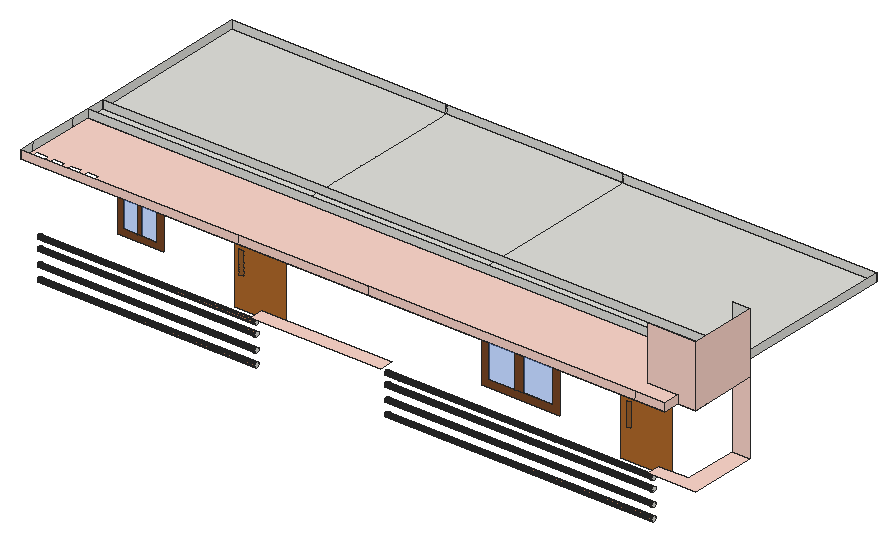
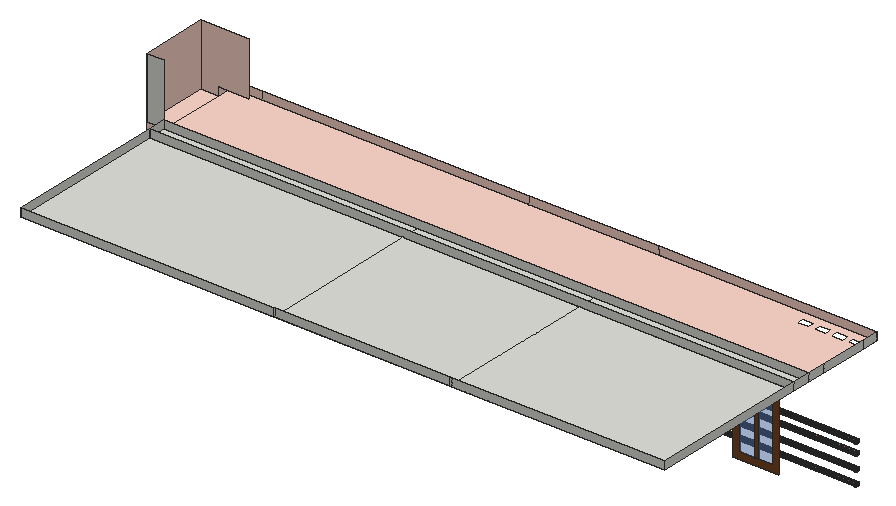
# SketchUp Ruby script. Lengths in inches.
U = 1.inch
M = Sketchup.active_model
def pt(a) = Geom::Point3d.new(a.map { |v| v * U })
def face(e, loops, mat)
  f = e.add_face(loops[0].map { |a| pt(a) })
  loops[1..].each { |l| e.add_face(l.map { |a| pt(a) }).erase! }
  f.material = f.back_material = mat if mat
  f
end
# faces: each face lists its corners as indices into pts; further lists are holes
def faces(e, pts, list, mat = nil) = list.each { |f| face(e, (f[0].is_a?(Array) ? f : [f]).map { |l| l.map { |i| pts[i] } }, mat) }
# xy, xz, yz: faces in a plane at the given z, y or x. An outline is a flat list of corners, or four numbers for a rectangle; further outlines are holes
def ring(l) = l.size == 4 ? [[l[0], l[1]], [l[2], l[1]], [l[2], l[3]], [l[0], l[3]]] : l.each_slice(2).to_a
def flat(e, list, mat, &to3) = list.each { |f| face(e, (f[0].is_a?(Array) ? f : [f]).map { |l| ring(l).map { |u, v| to3.(u, v) } }, mat) }
def xy(e, z, list, mat = nil) = flat(e, list, mat) { |x, y| [x, y, z] }
def xz(e, y, list, mat = nil) = flat(e, list, mat) { |x, z| [x, y, z] }
def yz(e, x, list, mat = nil) = flat(e, list, mat) { |y, z| [x, y, z] }
def lines(e, pts, list) = list.each { |a, b| e.add_line(pt(pts[a]), pt(pts[b])) }
# prism: a flat outline (further loops are holes) pulled along v
def prism(e, loops, v, mat = nil)
  f = face(e, loops, mat); d = Geom::Vector3d.new(v.map { |x| x * U })
  f.pushpull(f.normal.samedirection?(d) ? d.length : -d.length)
end
def box(e, o, s, mat = nil) = prism(e, [[o, [o[0] + s[0], o[1], o[2]], [o[0] + s[0], o[1] + s[1], o[2]], [o[0], o[1] + s[1], o[2]]]], [0, 0, s[2]], mat)
def at(x, y, z, deg = 0) = Geom::Transformation.translation(pt([x, y, z])) * Geom::Transformation.rotation(ORIGIN, Z_AXIS, deg.degrees)
def axes(o, x, y, z) = Geom::Transformation.new([*x, 0, *y, 0, *z, 0, *pt(o).to_a, 1])
def part(name) = M.definitions.add(name)
# library, detail: a bought-in or finely detailed component or shape, given as its bounding box
def library(name, o, s) = part(name).tap { |d| box(d.entities, o, s) }
def detail(e, o, s) = box(e.add_group.entities, o, s)
def put(e, d, t, mat = nil) = e.add_instance(d, t).tap { |i| i.material = mat if mat }
def group(e, t, mat = nil) = e.add_group.tap { |g| g.transformation = t; g.material = mat if mat }.entities
root = M.entities
M.materials.add("[Color B01]").color = [255, 216, 204]
M.materials.add("[Translucent Glass Blue]").color = [100, 149, 237]
M.materials["[Translucent Glass Blue]"].alpha = 0.5
M.materials.add("[Wood Bamboo]").color = [177, 105, 43]
M.materials.add("[Wood Floor Dark]").color = [153, 94, 42]
M.materials.add("[Wood Veneer 01]1").color = [120, 70, 37]
M.materials.add("[Wood Veneer 02]").color = [190, 128, 91]
xy(root,1559.8125,[[1696.31,288.33,1698.73,288.65,1700.99,289.59,1702.94,291.08,1704.43,293.02,1705.36,295.28,1705.68,297.71,1705.36,300.13,1704.43,302.39,1702.94,304.34,1700.99,305.83,1698.73,306.76,1696.31,307.08,1693.88,306.76,1691.62,305.83,1689.68,304.34,1688.1875,302.39,1687.25,300.13,1686.93,297.71,1687.25,295.28,1688.1875,293.02,1689.68,291.08,1691.62,289.59,1693.88,288.65]])
xy(root,1560.375,[[2395.24,288.33,2397.67,288.65,2399.93,289.59,2401.87,291.08,2403.36,293.02,2404.3,295.28,2404.62,297.71,2404.3,300.13,2403.36,302.39,2401.87,304.34,2399.93,305.83,2397.67,306.76,2395.24,307.08,2392.82,306.76,2390.56,305.83,2388.61,304.34,2387.125,302.39,2386.1875,300.13,2385.87,297.71,2386.1875,295.28,2387.125,293.02,2388.61,291.08,2390.56,289.59,2392.82,288.65]])
xy(root,1561,[[116.87,288.33,119.3,288.65,121.56,289.59,123.5,291.08,124.99,293.02,125.92,295.28,126.24,297.71,125.92,300.13,124.99,302.39,123.5,304.34,121.56,305.83,119.3,306.76,116.87,307.08,114.44,306.76,112.18,305.83,110.24,304.34,108.75,302.39,107.8125,300.13,107.49,297.71,107.8125,295.28,108.75,293.02,110.24,291.08,112.18,289.59,114.44,288.65]])
xy(root,1561.375,[[664.37,288.33,666.8,288.65,669.06,289.59,671,291.08,672.49,293.02,673.42,295.28,673.74,297.71,673.42,300.13,672.49,302.39,671,304.34,669.06,305.83,666.8,306.76,664.37,307.08,661.94,306.76,659.68,305.83,657.74,304.34,656.25,302.39,655.3125,300.13,654.99,297.71,655.3125,295.28,656.25,293.02,657.74,291.08,659.68,289.59,661.94,288.65]])
xy(root,1562.5625,[[2740.43,288.33,2742.86,288.65,2745.12,289.59,2747.06,291.08,2748.55,293.02,2749.49,295.28,2749.81,297.71,2749.49,300.13,2748.55,302.39,2747.06,304.34,2745.12,305.83,2742.86,306.76,2740.43,307.08,2738,306.76,2735.74,305.83,2733.8,304.34,2732.3125,302.39,2731.375,300.13,2731.06,297.71,2731.375,295.28,2732.3125,293.02,2733.8,291.08,2735.74,289.59,2738,288.65]])
xy(root,1563.22,[[984.12,288.33,986.55,288.65,988.81,289.59,989.8,290.35,978.43,290.35,979.43,289.59,981.69,288.65],[978.43,290.35,989.8,290.35,990.75,291.08,992.24,293.02,993.17,295.28,993.49,297.71,993.17,300.13,992.24,302.39,990.75,304.34,988.81,305.83,986.55,306.76,984.12,307.08,981.69,306.76,979.43,305.83,977.49,304.34,976,302.39,975.0625,300.13,974.74,297.71,975.0625,295.28,976,293.02,977.49,291.08]])
xy(root,1563.8125,[[2027.68,288.33,2030.11,288.65,2032.37,289.59,2034.31,291.08,2035.8,293.02,2036.74,295.28,2037.06,297.71,2036.74,300.13,2035.8,302.39,2034.31,304.34,2032.37,305.83,2030.11,306.76,2027.68,307.08,2025.25,306.76,2022.99,305.83,2021.05,304.34,2019.5625,302.39,2018.625,300.13,2018.31,297.71,2018.625,295.28,2019.5625,293.02,2021.05,291.08,2022.99,289.59,2025.25,288.65]])
xy(root,1564.4375,[[319.87,288.33,322.3,288.65,324.56,289.59,326.5,291.08,327.99,293.02,328.92,295.28,329.24,297.71,328.92,300.13,327.99,302.39,326.5,304.34,324.56,305.83,322.3,306.76,319.87,307.08,317.44,306.76,315.18,305.83,313.24,304.34,311.75,302.39,310.8125,300.13,310.49,297.71,310.8125,295.28,311.75,293.02,313.24,291.08,315.18,289.59,317.44,288.65]])
xy(root,1594.125,[[1053.15,267.5625,1631.4,328.8],[2829.41,267.5625,3040.15,267.5625,3040.15,571.9,2962.22,571.9,2962.22,328.8,2829.41,328.8]],"[Color B01]")
xy(root,1920.4375,[[77.93,571.9,1038.88,653.97],[1038.88,571.9,1828.6875,653.97],[1828.6875,571.9,2962.22,653.97],[77.93,653.97,1038.88,1377.24],[1038.88,653.97,1828.6875,1377.24],
  [1828.6875,653.97,2962.22,1377.24]])
xy(root,1920.4375,[[[77.93,195.0625,2962.22,571.9],[95.12,236.1875,148.18,267.5625],[170,236.1875,223.06,267.5625],[245.93,236.1875,299,267.5625],[321,236.1875,374.06,267.5625]],[2962.22,267.5625,3040.15,571.9]],"[Color B01]")
xz(root,195.0625,[[77.93,1920.4375,1053.15,1956.4375],[1053.15,1920.4375,1631.4,1956.4375],[1631.4,1920.4375,2829.41,1956.4375],[2829.41,1920.4375,2962.22,1956.4375]],"[Color B01]")
xz(root,267.5625,[[2962.22,1920.4375,3040.15,1920.4375,3040.15,2195.8125,2829.41,2195.8125,2829.41,1956.4375,2962.22,1956.4375]],"[Color B01]")
xz(root,571.9,[[77.93,1920.4375,2962.22,1956.4375],[2962.22,1920.4375,3040.15,2195.8125]])
xz(root,571.9,[[2962.22,1594.125,3040.15,1920.4375]],"[Color B01]")
xz(root,571.9,[[1871.31,1500.05,1989.8125,1788.37],[2027.45,1500.05,2159.625,1788.37],[239.7,1528.97,301.71,1805.47],[318.375,1528.97,388.8125,1805.47]],"[Translucent Glass Blue]")
xz(root,571.9,[[[2462.81,1393.34,2689.8125,1805.49],[2489.37,1528.97,2509.1,1632.89]],[[735.89,1393.5,966.45,1811.59],[755.24,1528.97,774.97,1632.89]]],"[Wood Bamboo]")
xz(root,571.9,[[755.24,1528.97,774.97,1632.89],[2489.37,1528.97,2509.1,1632.89]],"[Wood Floor Dark]")
xz(root,571.9,[[[1839.4375,1468.18,2191.5,1820.24],[1871.31,1500.05,2159.625,1788.37]],[1989.8125,1500.05,2027.45,1788.37],[[211.19,1500.46,417.32,1833.98],[239.7,1528.97,388.8125,1805.47]],[301.71,1528.97,318.375,1805.47]],"[Wood Veneer 01]1")
xz(root,653.97,[[77.93,1920.4375,2962.22,1956.4375]])
xz(root,1377.24,[[77.93,1920.4375,1031.89,1956.4375],[1031.89,1920.4375,1038.88,1956.4375],[1038.88,1920.4375,1822.57,1956.4375],[1822.57,1920.4375,1828.6875,1956.4375],[1828.6875,1920.4375,2962.22,1956.4375]])
yz(root,77.93,[[195.0625,1920.4375,267.5625,1956.4375],[267.5625,1920.4375,488.625,1956.4375],[488.625,1920.4375,571.9,1956.4375],[571.9,1920.4375,653.97,1956.4375],[653.97,1920.4375,1377.24,1956.4375]])
yz(root,1053.15,[[299.67,1381.78,302.08,1382.1,304.32,1383.03,306.25,1384.51,307.73,1386.4375,308.66,1388.68,308.98,1391.09,308.66,1393.5,307.73,1395.75,306.25,1397.68,304.32,1399.16,302.08,1400.09,299.67,1400.41,297.25,1400.09,295.01,1399.16,293.08,1397.68,291.6,1395.75,290.67,1393.5,290.35,1391.09,290.67,1388.68,291.6,1386.4375,293.08,1384.51,295.01,1383.03,297.25,1382.1],[299.67,1440.84,302.08,1441.16,304.32,1442.09,306.25,1443.57,307.73,1445.5,308.66,1447.74,308.98,1450.16,308.66,1452.57,307.73,1454.8125,306.25,1456.74,304.32,1458.22,302.08,1459.15,299.67,1459.47,297.25,1459.15,295.01,1458.22,293.08,1456.74,291.6,1454.8125,290.67,1452.57,290.35,1450.16,290.67,1447.74,291.6,1445.5,293.08,1443.57,295.01,1442.09,297.25,1441.16],[299.67,1504.28,302.08,1504.6,304.32,1505.53,306.25,1507.01,307.73,1508.9375,308.66,1511.18,308.98,1513.59,308.66,1516,307.73,1518.25,306.25,1520.18,304.32,1521.66,302.08,1522.59,299.67,1522.91,297.25,1522.59,295.01,1521.66,293.08,1520.18,291.6,1518.25,290.67,1516,290.35,1513.59,290.67,1511.18,291.6,1508.9375,293.08,1507.01,295.01,1505.53,297.25,1504.6],[299.67,1553.91,302.08,1554.22,304.32,1555.15,306.25,1556.63,307.73,1558.5625,308.66,1560.81,308.98,1563.22,308.66,1565.63,307.73,1567.875,306.25,1569.8,304.32,1571.28,302.08,1572.21,299.67,1572.53,297.25,1572.21,295.01,1571.28,293.08,1569.8,291.6,1567.875,290.67,1565.63,290.35,1563.22,290.67,1560.81,291.6,1558.5625,293.08,1556.63,295.01,1555.15,297.25,1554.22]])
yz(root,2829.41,[[299.67,1388.28,302.08,1388.6,304.32,1389.53,306.25,1391.01,307.73,1392.9375,308.66,1395.18,308.98,1397.59,308.66,1400,307.73,1402.25,306.25,1404.18,304.32,1405.66,302.08,1406.59,299.67,1406.91,297.25,1406.59,295.01,1405.66,293.08,1404.18,291.6,1402.25,290.67,1400,290.35,1397.59,290.67,1395.18,291.6,1392.9375,293.08,1391.01,295.01,1389.53,297.25,1388.6],[299.67,1445.16,302.08,1445.47,304.32,1446.4,306.25,1447.88,307.73,1449.8125,308.66,1452.06,308.98,1454.47,308.66,1456.88,307.73,1459.125,306.25,1461.05,304.32,1462.53,302.08,1463.46,299.67,1463.78,297.25,1463.46,295.01,1462.53,293.08,1461.05,291.6,1459.125,290.67,1456.88,290.35,1454.47,290.67,1452.06,291.6,1449.8125,293.08,1447.88,295.01,1446.4,297.25,1445.47],[299.67,1507.03,302.08,1507.35,304.32,1508.28,306.25,1509.76,307.73,1511.6875,308.66,1513.93,308.98,1516.34,308.66,1518.75,307.73,1521,306.25,1522.93,304.32,1524.41,302.08,1525.34,299.67,1525.66,297.25,1525.34,295.01,1524.41,293.08,1522.93,291.6,1521,290.67,1518.75,290.35,1516.34,290.67,1513.93,291.6,1511.6875,293.08,1509.76,295.01,1508.28,297.25,1507.35],[299.67,1553.91,302.08,1554.22,304.32,1555.15,306.25,1556.63,307.73,1558.5625,308.66,1560.81,308.98,1563.22,308.66,1565.63,307.73,1567.875,306.25,1569.8,304.32,1571.28,302.08,1572.21,299.67,1572.53,297.25,1572.21,295.01,1571.28,293.08,1569.8,291.6,1567.875,290.67,1565.63,290.35,1563.22,290.67,1560.81,291.6,1558.5625,293.08,1556.63,295.01,1555.15,297.25,1554.22]])
yz(root,2962.22,[[571.9,1920.4375,653.97,1956.4375],[653.97,1920.4375,1377.24,1956.4375]])
yz(root,2962.22,[[195.0625,1920.4375,267.5625,1956.4375]],"[Color B01]")
yz(root,3040.15,[[267.5625,1920.4375,571.9,2195.8125]],"[Color B01]")
p = [[1053.15,299.67,1381.78],[1053.15,297.25,1382.1],[77.93,297.25,1382.1],[77.93,299.67,1381.78],[1053.15,302.08,1382.1],[77.93,302.08,1382.1],
  [1053.15,295.01,1383.03],[77.93,295.01,1383.03],[1053.15,304.32,1383.03],[77.93,304.32,1383.03],[1053.15,293.08,1384.51],[77.93,293.08,1384.51],
  [1053.15,306.25,1384.51],[77.93,306.25,1384.51],[1053.15,291.6,1386.4375],[77.93,291.6,1386.4375],[1053.15,307.73,1386.4375],[77.93,307.73,1386.4375],
  [1053.15,290.67,1388.68],[77.93,290.67,1388.68],[1053.15,308.66,1388.68],[77.93,308.66,1388.68],[2829.41,299.67,1388.28],[2829.41,297.25,1388.6],
  [1631.4,297.25,1388.6],[1631.4,299.67,1388.28],[2829.41,302.08,1388.6],[1631.4,302.08,1388.6],[2829.41,295.01,1389.53],[1631.4,295.01,1389.53],
  [2829.41,304.32,1389.53],[1631.4,304.32,1389.53],[1053.15,290.35,1391.09],[77.93,290.35,1391.09],[1053.15,308.98,1391.09],[77.93,308.98,1391.09],
  [2829.41,293.08,1391.01],[1631.4,293.08,1391.01],[2829.41,306.25,1391.01],[1631.4,306.25,1391.01],[2829.41,291.6,1392.9375],[1631.4,291.6,1392.9375],
  [2829.41,307.73,1392.9375],[1631.4,307.73,1392.9375],[1053.15,290.67,1393.5],[77.93,290.67,1393.5],[1053.15,308.66,1393.5],[77.93,308.66,1393.5],
  [2829.41,290.67,1395.18],[1631.4,290.67,1395.18],[2829.41,308.66,1395.18],[1631.4,308.66,1395.18],[1053.15,291.6,1395.75],[77.93,291.6,1395.75],
  [1053.15,307.73,1395.75],[77.93,307.73,1395.75],[2829.41,290.35,1397.59],[1631.4,290.35,1397.59],[2829.41,308.98,1397.59],[1631.4,308.98,1397.59],
  [1053.15,293.08,1397.68],[77.93,293.08,1397.68],[1053.15,306.25,1397.68],[77.93,306.25,1397.68],[2829.41,290.67,1400],[1631.4,290.67,1400],
  [2829.41,308.66,1400],[1631.4,308.66,1400],[1053.15,295.01,1399.16],[77.93,295.01,1399.16],[1053.15,304.32,1399.16],[77.93,304.32,1399.16],
  [1053.15,297.25,1400.09],[77.93,297.25,1400.09],[1053.15,302.08,1400.09],[77.93,302.08,1400.09],[2829.41,291.6,1402.25],[1631.4,291.6,1402.25],
  [2829.41,307.73,1402.25],[1631.4,307.73,1402.25],[1053.15,299.67,1400.41],[77.93,299.67,1400.41],[2829.41,293.08,1404.18],[1631.4,293.08,1404.18],
  [2829.41,306.25,1404.18],[1631.4,306.25,1404.18],[2829.41,295.01,1405.66],[1631.4,295.01,1405.66],[2829.41,304.32,1405.66],[1631.4,304.32,1405.66],
  [2829.41,297.25,1406.59],[1631.4,297.25,1406.59],[2829.41,302.08,1406.59],[1631.4,302.08,1406.59],[2829.41,299.67,1406.91],[1631.4,299.67,1406.91],
  [1053.15,299.67,1440.84],[1053.15,297.25,1441.16],[77.93,297.25,1441.16],[77.93,299.67,1440.84],[1053.15,302.08,1441.16],[77.93,302.08,1441.16],
  [1053.15,295.01,1442.09],[77.93,295.01,1442.09],[1053.15,304.32,1442.09],[77.93,304.32,1442.09],[1053.15,293.08,1443.57],[77.93,293.08,1443.57],
  [1053.15,306.25,1443.57],[77.93,306.25,1443.57],[1053.15,291.6,1445.5],[77.93,291.6,1445.5],[1053.15,307.73,1445.5],[77.93,307.73,1445.5],
  [2829.41,299.67,1445.16],[2829.41,297.25,1445.47],[1631.4,297.25,1445.47],[1631.4,299.67,1445.16],[2829.41,302.08,1445.47],[1631.4,302.08,1445.47],
  [1053.15,290.67,1447.74],[77.93,290.67,1447.74],[2829.41,295.01,1446.4],[1631.4,295.01,1446.4],[2829.41,304.32,1446.4],[1631.4,304.32,1446.4],
  [1053.15,308.66,1447.74],[77.93,308.66,1447.74],[2829.41,293.08,1447.88],[1631.4,293.08,1447.88],[2829.41,306.25,1447.88],[1631.4,306.25,1447.88],
  [1053.15,290.35,1450.16],[77.93,290.35,1450.16],[1053.15,308.98,1450.16],[77.93,308.98,1450.16],[2829.41,291.6,1449.8125],[1631.4,291.6,1449.8125],
  [2829.41,307.73,1449.8125],[1631.4,307.73,1449.8125],[2829.41,290.67,1452.06],[1631.4,290.67,1452.06],[2829.41,308.66,1452.06],[1631.4,308.66,1452.06],
  [1053.15,290.67,1452.57],[77.93,290.67,1452.57],[1053.15,308.66,1452.57],[77.93,308.66,1452.57],[2829.41,290.35,1454.47],[1631.4,290.35,1454.47],
  [2829.41,308.98,1454.47],[1631.4,308.98,1454.47],[1053.15,291.6,1454.8125],[77.93,291.6,1454.8125],[1053.15,307.73,1454.8125],[77.93,307.73,1454.8125],
  [2829.41,290.67,1456.88],[1631.4,290.67,1456.88],[2829.41,308.66,1456.88],[1631.4,308.66,1456.88],[1053.15,293.08,1456.74],[77.93,293.08,1456.74],
  [1053.15,306.25,1456.74],[77.93,306.25,1456.74],[1053.15,295.01,1458.22],[77.93,295.01,1458.22],[1053.15,304.32,1458.22],[77.93,304.32,1458.22],
  [2829.41,291.6,1459.125],[1631.4,291.6,1459.125],[2829.41,307.73,1459.125],[1631.4,307.73,1459.125],[1053.15,297.25,1459.15],[77.93,297.25,1459.15],
  [1053.15,302.08,1459.15],[77.93,302.08,1459.15],[2829.41,293.08,1461.05],[1631.4,293.08,1461.05],[2829.41,306.25,1461.05],[1631.4,306.25,1461.05],
  [1053.15,299.67,1459.47],[77.93,299.67,1459.47],[2829.41,295.01,1462.53],[1631.4,295.01,1462.53],[2829.41,304.32,1462.53],[1631.4,304.32,1462.53],
  [2829.41,297.25,1463.46],[1631.4,297.25,1463.46],[2829.41,302.08,1463.46],[1631.4,302.08,1463.46],[2829.41,299.67,1463.78],[1631.4,299.67,1463.78],
  [1053.15,299.67,1504.28],[1053.15,297.25,1504.6],[77.93,297.25,1504.6],[77.93,299.67,1504.28],[1053.15,302.08,1504.6],[77.93,302.08,1504.6],
  [1053.15,295.01,1505.53],[77.93,295.01,1505.53],[1053.15,304.32,1505.53],[77.93,304.32,1505.53],[1053.15,293.08,1507.01],[77.93,293.08,1507.01],
  [1053.15,306.25,1507.01],[77.93,306.25,1507.01],[1053.15,291.6,1508.9375],[77.93,291.6,1508.9375],[2829.41,299.67,1507.03],[2829.41,297.25,1507.35],
  [1631.4,297.25,1507.35],[1631.4,299.67,1507.03],[2829.41,302.08,1507.35],[1631.4,302.08,1507.35],[1053.15,307.73,1508.9375],[77.93,307.73,1508.9375],
  [2829.41,295.01,1508.28],[1631.4,295.01,1508.28],[2829.41,304.32,1508.28],[1631.4,304.32,1508.28],[2829.41,293.08,1509.76],[1631.4,293.08,1509.76],
  [2829.41,306.25,1509.76],[1631.4,306.25,1509.76],[1053.15,290.67,1511.18],[77.93,290.67,1511.18],[1053.15,308.66,1511.18],[77.93,308.66,1511.18],
  [2829.41,291.6,1511.6875],[1631.4,291.6,1511.6875],[2829.41,307.73,1511.6875],[1631.4,307.73,1511.6875],[1053.15,290.35,1513.59],[77.93,290.35,1513.59],
  [1053.15,308.98,1513.59],[77.93,308.98,1513.59],[2829.41,290.67,1513.93],[1631.4,290.67,1513.93],[2829.41,308.66,1513.93],[1631.4,308.66,1513.93],
  [1053.15,290.67,1516],[77.93,290.67,1516],[1053.15,308.66,1516],[77.93,308.66,1516],[2829.41,290.35,1516.34],[1631.4,290.35,1516.34],
  [2829.41,308.98,1516.34],[1631.4,308.98,1516.34],[1053.15,291.6,1518.25],[77.93,291.6,1518.25],[1053.15,307.73,1518.25],[77.93,307.73,1518.25],
  [2829.41,290.67,1518.75],[1631.4,290.67,1518.75],[2829.41,308.66,1518.75],[1631.4,308.66,1518.75],[1053.15,293.08,1520.18],[77.93,293.08,1520.18],
  [1053.15,306.25,1520.18],[77.93,306.25,1520.18],[2829.41,291.6,1521],[1631.4,291.6,1521],[2829.41,307.73,1521],[1631.4,307.73,1521],
  [1053.15,295.01,1521.66],[77.93,295.01,1521.66],[1053.15,304.32,1521.66],[77.93,304.32,1521.66],[2829.41,293.08,1522.93],[1631.4,293.08,1522.93],
  [2829.41,306.25,1522.93],[1631.4,306.25,1522.93],[1053.15,297.25,1522.59],[77.93,297.25,1522.59],[1053.15,302.08,1522.59],[77.93,302.08,1522.59],
  [1053.15,299.67,1522.91],[77.93,299.67,1522.91],[2829.41,295.01,1524.41],[1631.4,295.01,1524.41],[2829.41,304.32,1524.41],[1631.4,304.32,1524.41],
  [2829.41,297.25,1525.34],[1631.4,297.25,1525.34],[2829.41,302.08,1525.34],[1631.4,302.08,1525.34],[2829.41,299.67,1525.66],[1631.4,299.67,1525.66],
  [1053.15,299.67,1553.91],[1053.15,297.25,1554.22],[77.93,297.25,1554.22],[77.93,299.67,1553.91],[2829.41,299.67,1553.91],[2829.41,297.25,1554.22],
  [1631.4,297.25,1554.22],[1631.4,299.67,1553.91],[1053.15,302.08,1554.22],[77.93,302.08,1554.22],[2829.41,302.08,1554.22],[1631.4,302.08,1554.22],
  [1053.15,295.01,1555.15],[77.93,295.01,1555.15],[2829.41,295.01,1555.15],[1631.4,295.01,1555.15],[1053.15,304.32,1555.15],[77.93,304.32,1555.15],
  [2829.41,304.32,1555.15],[1631.4,304.32,1555.15],[1053.15,293.08,1556.63],[77.93,293.08,1556.63],[2829.41,293.08,1556.63],[1631.4,293.08,1556.63],
  [1053.15,306.25,1556.63],[77.93,306.25,1556.63],[2829.41,306.25,1556.63],[1631.4,306.25,1556.63],[1053.15,291.6,1558.5625],[77.93,291.6,1558.5625],
  [2829.41,291.6,1558.5625],[1631.4,291.6,1558.5625],[1053.15,307.73,1558.5625],[77.93,307.73,1558.5625],[2829.41,307.73,1558.5625],[1631.4,307.73,1558.5625],
  [1053.15,290.67,1560.81],[77.93,290.67,1560.81],[2829.41,290.67,1560.81],[1631.4,290.67,1560.81],[1053.15,308.66,1560.81],[77.93,308.66,1560.81],
  [2829.41,308.66,1560.81],[1631.4,308.66,1560.81],[1053.15,290.35,1563.22],[989.8,290.35,1563.22],[978.43,290.35,1563.22],[77.93,290.35,1563.22],
  [2829.41,290.35,1563.22],[1631.4,290.35,1563.22],[1053.15,308.98,1563.22],[77.93,308.98,1563.22],[2829.41,308.98,1563.22],[1631.4,308.98,1563.22],
  [1053.15,290.67,1565.63],[77.93,290.67,1565.63],[2829.41,290.67,1565.63],[1631.4,290.67,1565.63],[1053.15,308.66,1565.63],[77.93,308.66,1565.63],
  [2829.41,308.66,1565.63],[1631.4,308.66,1565.63],[1053.15,291.6,1567.875],[77.93,291.6,1567.875],[2829.41,291.6,1567.875],[1631.4,291.6,1567.875],
  [1053.15,307.73,1567.875],[77.93,307.73,1567.875],[2829.41,307.73,1567.875],[1631.4,307.73,1567.875],[1053.15,293.08,1569.8],[77.93,293.08,1569.8],
  [2829.41,293.08,1569.8],[1631.4,293.08,1569.8],[1053.15,306.25,1569.8],[77.93,306.25,1569.8],[2829.41,306.25,1569.8],[1631.4,306.25,1569.8],
  [1053.15,295.01,1571.28],[77.93,295.01,1571.28],[2829.41,295.01,1571.28],[1631.4,295.01,1571.28],[1053.15,304.32,1571.28],[77.93,304.32,1571.28],
  [2829.41,304.32,1571.28],[1631.4,304.32,1571.28],[1053.15,297.25,1572.21],[77.93,297.25,1572.21],[2829.41,297.25,1572.21],[1631.4,297.25,1572.21],
  [1053.15,302.08,1572.21],[77.93,302.08,1572.21],[2829.41,302.08,1572.21],[1631.4,302.08,1572.21],[1053.15,299.67,1572.53],[77.93,299.67,1572.53],
  [2829.41,299.67,1572.53],[1631.4,299.67,1572.53],[3040.15,328.8,1920.4375],[3040.27,328.8,1920.4375]]
faces(root,p,[[0,1,2,3],[4,0,3,5],[1,6,7,2],[8,4,5,9],[6,10,11,7],[12,8,9,13],[10,14,15,11],[16,12,13,17],
  [14,18,19,15],[20,16,17,21],[22,23,24,25],[26,22,25,27],[23,28,29,24],[30,26,27,31],[18,32,33,19],[34,20,21,35],
  [28,36,37,29],[38,30,31,39],[36,40,41,37],[42,38,39,43],[32,44,45,33],[46,34,35,47],[40,48,49,41],[50,42,43,51],
  [44,52,53,45],[54,46,47,55],[48,56,57,49],[58,50,51,59],[52,60,61,53],[62,54,55,63],[56,64,65,57],[66,58,59,67],
  [60,68,69,61],[70,62,63,71],[68,72,73,69],[74,70,71,75],[64,76,77,65],[78,66,67,79],[72,80,81,73],[80,74,75,81],
  [76,82,83,77],[84,78,79,85],[82,86,87,83],[88,84,85,89],[86,90,91,87],[92,88,89,93],[90,94,95,91],[94,92,93,95],
  [96,97,98,99],[100,96,99,101],[97,102,103,98],[104,100,101,105],[102,106,107,103],[108,104,105,109],[106,110,111,107],[112,108,109,113],
  [114,115,116,117],[118,114,117,119],[110,120,121,111],[115,122,123,116],[124,118,119,125],[126,112,113,127],[122,128,129,123],[130,124,125,131],
  [120,132,133,121],[134,126,127,135],[128,136,137,129],[138,130,131,139],[136,140,141,137],[142,138,139,143],[132,144,145,133],[146,134,135,147],
  [140,148,149,141],[150,142,143,151],[144,152,153,145],[154,146,147,155],[148,156,157,149],[158,150,151,159],[152,160,161,153],[162,154,155,163],
  [160,164,165,161],[166,162,163,167],[156,168,169,157],[170,158,159,171],[164,172,173,165],[174,166,167,175],[168,176,177,169],[178,170,171,179],
  [172,180,181,173],[180,174,175,181],[176,182,183,177],[184,178,179,185],[182,186,187,183],[188,184,185,189],[186,190,191,187],[190,188,189,191],
  [192,193,194,195],[196,192,195,197],[193,198,199,194],[200,196,197,201],[198,202,203,199],[204,200,201,205],[202,206,207,203],[208,209,210,211],
  [212,208,211,213],[214,204,205,215],[209,216,217,210],[218,212,213,219],[216,220,221,217],[222,218,219,223],[206,224,225,207],[226,214,215,227],
  [220,228,229,221],[230,222,223,231],[224,232,233,225],[234,226,227,235],[228,236,237,229],[238,230,231,239],[232,240,241,233],[242,234,235,243],
  [236,244,245,237],[246,238,239,247],[240,248,249,241],[250,242,243,251],[244,252,253,245],[254,246,247,255],[248,256,257,249],[258,250,251,259],
  [252,260,261,253],[262,254,255,263],[256,264,265,257],[266,258,259,267],[260,268,269,261],[270,262,263,271],[264,272,273,265],[274,266,267,275],
  [272,276,277,273],[276,274,275,277],[268,278,279,269],[280,270,271,281],[278,282,283,279],[284,280,281,285],[282,286,287,283],[286,284,285,287],
  [288,289,290,291],[292,293,294,295],[296,288,291,297],[298,292,295,299],[289,300,301,290],[293,302,303,294],[304,296,297,305],[306,298,299,307],
  [300,308,309,301],[302,310,311,303],[312,304,305,313],[314,306,307,315],[308,316,317,309],[310,318,319,311],[320,312,313,321],[322,314,315,323],
  [316,324,325,317],[318,326,327,319],[328,320,321,329],[330,322,323,331],[324,332,333,334,335,325],[326,336,337,327],[338,328,329,339],[340,330,331,341],
  [332,342,343,335,334,333],[336,344,345,337],[346,338,339,347],[348,340,341,349],[342,350,351,343],[344,352,353,345],[354,346,347,355],[356,348,349,357],
  [350,358,359,351],[352,360,361,353],[362,354,355,363],[364,356,357,365],[358,366,367,359],[360,368,369,361],[370,362,363,371],[372,364,365,373],
  [366,374,375,367],[368,376,377,369],[378,370,371,379],[380,372,373,381],[374,382,383,375],[376,384,385,377],[382,378,379,383],[384,380,381,385]],"[Wood Veneer 02]")
lines(root,p,[[386,387]])
